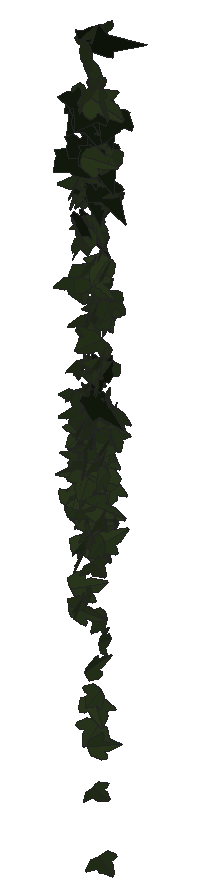
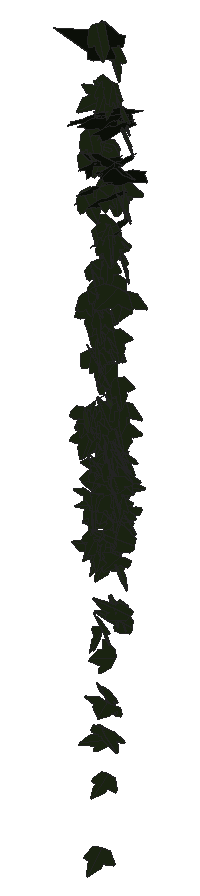
# SketchUp Ruby script. Lengths in inches.
U = 1.inch
M = Sketchup.active_model
def pt(a) = Geom::Point3d.new(a.map { |v| v * U })
def face(e, loops, mat)
  f = e.add_face(loops[0].map { |a| pt(a) })
  loops[1..].each { |l| e.add_face(l.map { |a| pt(a) }).erase! }
  f.material = f.back_material = mat if mat
  f
end
# faces: each face lists its corners as indices into pts; further lists are holes
def faces(e, pts, list, mat = nil) = list.each { |f| face(e, (f[0].is_a?(Array) ? f : [f]).map { |l| l.map { |i| pts[i] } }, mat) }
# xy, xz, yz: faces in a plane at the given z, y or x. An outline is a flat list of corners, or four numbers for a rectangle; further outlines are holes
def ring(l) = l.size == 4 ? [[l[0], l[1]], [l[2], l[1]], [l[2], l[3]], [l[0], l[3]]] : l.each_slice(2).to_a
def flat(e, list, mat, &to3) = list.each { |f| face(e, (f[0].is_a?(Array) ? f : [f]).map { |l| ring(l).map { |u, v| to3.(u, v) } }, mat) }
def xy(e, z, list, mat = nil) = flat(e, list, mat) { |x, y| [x, y, z] }
def xz(e, y, list, mat = nil) = flat(e, list, mat) { |x, z| [x, y, z] }
def yz(e, x, list, mat = nil) = flat(e, list, mat) { |y, z| [x, y, z] }
def lines(e, pts, list) = list.each { |a, b| e.add_line(pt(pts[a]), pt(pts[b])) }
# prism: a flat outline (further loops are holes) pulled along v
def prism(e, loops, v, mat = nil)
  f = face(e, loops, mat); d = Geom::Vector3d.new(v.map { |x| x * U })
  f.pushpull(f.normal.samedirection?(d) ? d.length : -d.length)
end
def box(e, o, s, mat = nil) = prism(e, [[o, [o[0] + s[0], o[1], o[2]], [o[0] + s[0], o[1] + s[1], o[2]], [o[0], o[1] + s[1], o[2]]]], [0, 0, s[2]], mat)
def at(x, y, z, deg = 0) = Geom::Transformation.translation(pt([x, y, z])) * Geom::Transformation.rotation(ORIGIN, Z_AXIS, deg.degrees)
def axes(o, x, y, z) = Geom::Transformation.new([*x, 0, *y, 0, *z, 0, *pt(o).to_a, 1])
def part(name) = M.definitions.add(name)
# library, detail: a bought-in or finely detailed component or shape, given as its bounding box
def library(name, o, s) = part(name).tap { |d| box(d.entities, o, s) }
def detail(e, o, s) = box(e.add_group.entities, o, s)
def put(e, d, t, mat = nil) = e.add_instance(d, t).tap { |i| i.material = mat if mat }
def group(e, t, mat = nil) = e.add_group.tap { |g| g.transformation = t; g.material = mat if mat }.entities
root = M.entities
M.materials.add("1026 AP 7946 SUNNY SIDE UP").color = [254, 231, 186]
M.materials.add("efeu1").color = [18, 25, 13]
M.materials.add("efeu2").color = [43, 57, 29]
c1 = part("ivyleaf_10")
p = [[0,0.5,-0.03],[-0.0625,2.02,-0.43],[-0.19,2.01,-0.46],[-0.54,1.05,-0.29],[-0.52,0.625,-0.18],[-0.83,0.76,-0.28],
  [-1.16,0.64,-0.33],[-1.15,0.33,-0.24],[-0.77,-0.39,0.02],[-0.3,-0.51,0.16],[0.04,-0.48,0.23],[-0.02,2.01,-0.4375],
  [-0.06,2.01,-0.43],[0.04,-0.49,0.23],[0.67,-0.49,0.14],[1.38,0.36,-0.2],[1.375,0.51,-0.24],[0.81,0.65,-0.19],
  [0.62,0.59,-0.15],[0.6,1.09,-0.28],[0.5,1.23,-0.31]]
faces(c1.entities,p,[[0,1,2,3,4,5,6,7,8,9,10],[11,12,0,13,14,15,16,17,18,19,20]],"efeu2")
c2 = part("ivyleaf_9")
p = [[1.54,2.16,1.25],[1.36,2.04,1.19],[-0.21,0.99,0.68],[-0.71,1.11,0.82],[-0.85,0.86,0.67],[-0.8,0.17,0.21],
  [-0.9,-0.01,0.1],[-0.67,-0.16,-0.02],[-0.08,-0.08,-0.05],[-0.03,-0.6,-0.4],[0.65,-0.88,-0.66],[0.83,-0.6,-0.49],
  [1.29,-0.42,-0.43],[1.8125,-0.07,-0.26],[1.21,0.44,0.15]]
faces(c2.entities,p,[[0,1,2,3,4,5,6,7,8,9,10,11,12,13,14]],"efeu1")
put(root,c1,axes([103.23,212.84,260.54],[-0.04694,-0.21641,-0.02736],[0.01178,0.02453,-0.22487],[0.3424,-0.03051,0.00399]),"1026 AP 7946 SUNNY SIDE UP")
put(root,c1,axes([103.25,212.84,259.06],[0.29938,-0.04666,-0.06917],[-0.11097,-0.00919,-0.20044],[0.06425,0.20159,-0.0239]),"1026 AP 7946 SUNNY SIDE UP")
put(root,c1,axes([103.31,212.77,258.55],[-0.28898,-0.07122,0.07311],[-0.08414,-0.05686,-0.20074],[0.13437,-0.18877,0.03152]),"1026 AP 7946 SUNNY SIDE UP")
put(root,c1,axes([103.3,212.68,263.19],[0.10199,-0.17927,-0.14312],[-0.09887,0.12352,-0.19515],[0.34162,0.08927,-0.01375]),"1026 AP 7946 SUNNY SIDE UP")
put(root,c1,axes([103.36,212.76,258.35],[0.02537,0.05885,-0.20622],[-0.24822,-0.12834,-0.05264],[-0.2153,0.1549,0.03639]),"1026 AP 7946 SUNNY SIDE UP")
put(root,c1,axes([103.25,212.75,259.54],[-0.16245,-0.19473,-0.00339],[0.01423,-0.00233,-0.22692],[0.30588,-0.10331,0.00875]),"1026 AP 7946 SUNNY SIDE UP")
put(root,c1,axes([103.28,212.8,258.09],[-0.26935,0.10482,0.02808],[-0.06448,-0.01673,-0.20375],[-0.15737,-0.17255,0.03542]),"1026 AP 7946 SUNNY SIDE UP")
put(root,c1,axes([103.26,212.6875,265.87],[0.2084,-0.21154,0.00222],[-0.01069,-0.00822,-0.257],[0.3325,0.13233,-0.00966]),"1026 AP 7946 SUNNY SIDE UP")
put(root,c1,axes([103.28,212.79,259.97],[-0.0656,-0.21468,-0.0423],[0.01333,0.03894,-0.22507],[0.34307,-0.04256,0.00066]),"1026 AP 7946 SUNNY SIDE UP")
put(root,c1,axes([103.24,212.68,262.31],[-0.2747,-0.15795,-0.04725],[0.07993,0.01042,-0.2411],[0.24556,-0.1801,0.02562]),"1026 AP 7946 SUNNY SIDE UP")
put(root,c1,axes([103.09,212.68,257.49],[0.16738,-0.12715,-0.14429],[0.16606,-0.0924,0.16944],[-0.24577,-0.14903,0.01622]),"1026 AP 7946 SUNNY SIDE UP")
put(root,c1,axes([103.3,212.59,264.51],[0.08272,-0.20959,-0.12985],[-0.0151,0.12585,-0.22107],[0.38331,0.05019,0.01931]),"1026 AP 7946 SUNNY SIDE UP")
put(root,c1,axes([103.26,212.86,259.22],[0.24489,-0.14597,0.00716],[-0.00431,-0.01428,-0.21961],[0.2298,0.15528,-0.01175]),"1026 AP 7946 SUNNY SIDE UP")
put(root,c1,axes([103.28,212.92,258.3],[0.1378,-0.1884,-0.00771],[0.00619,0.0089,-0.21388],[0.29635,0.08742,0.00805]),"1026 AP 7946 SUNNY SIDE UP")
put(root,c1,axes([103.4375,212.64,257.45],[0.25046,0.01853,0.16684],[-0.2547,0.04211,0.15951],[-0.02727,-0.22314,0.0426]),"1026 AP 7946 SUNNY SIDE UP")
put(root,c1,axes([103.27,212.9375,258.55],[0.27222,0.10499,-0.03679],[-0.04015,-0.02782,-0.20848],[-0.17,0.17469,-0.00967]),"1026 AP 7946 SUNNY SIDE UP")
put(root,c1,axes([103.3,212.72,257.41],[0.02496,-0.13732,-0.15549],[0.03087,0.15094,-0.13918],[0.31845,-0.00387,0.02568]),"1026 AP 7946 SUNNY SIDE UP")
put(root,c1,axes([103.05,212.86,257.27],[-0.03544,-0.04086,0.21982],[0.30269,0.0962,0.04044],[-0.15915,0.19206,0.02796]),"1026 AP 7946 SUNNY SIDE UP")
put(root,c1,axes([103.34,212.84,261.51],[-0.08217,-0.2236,0.00077],[0.00929,-0.00345,-0.23648],[0.35147,-0.05218,0.00643]),"1026 AP 7946 SUNNY SIDE UP")
put(root,c1,axes([103.3,212.68,257.78],[-0.10332,-0.18021,-0.08267],[0.06733,0.06844,-0.19656],[0.30212,-0.07688,0.01553]),"1026 AP 7946 SUNNY SIDE UP")
put(root,c1,axes([103.35,212.91,258.07],[-0.19602,-0.1599,0.04195],[0.01694,-0.05991,-0.20415],[0.25925,-0.11698,0.04506]),"1026 AP 7946 SUNNY SIDE UP")
put(root,c1,axes([103.35,212.67,266.32],[0.23053,-0.21398,-0.0296],[-0.02705,0.02157,-0.26709],[0.33816,0.1476,-0.00118]),"1026 AP 7946 SUNNY SIDE UP")
put(root,c1,axes([103.34,212.7,256.55],[0.11049,-0.19207,0.01732],[-0.00044,-0.01916,-0.21069],[0.30332,0.06994,-0.00661]),"1026 AP 7946 SUNNY SIDE UP")
put(root,c1,axes([103.34,212.67,264.38],[0.1732,-0.21768,0.02966],[0.00142,-0.03314,-0.2511],[0.34551,0.10926,-0.01384]),"1026 AP 7946 SUNNY SIDE UP")
put(root,c1,axes([103.36,212.63,259.94],[-0.34273,-0.04165,-0.0023],[0.00945,-0.02088,-0.22764],[0.06488,-0.21697,0.02102]),"1026 AP 7946 SUNNY SIDE UP")
put(root,c1,axes([103.27,212.5625,257.7],[0.24662,0.11259,-0.06619],[0.06847,0.0503,0.19862],[0.19253,-0.16212,0.01415]),"1026 AP 7946 SUNNY SIDE UP")
put(root,c1,axes([103.38,212.9,258.76],[-0.07272,-0.1991,0.054],[0.0002,-0.0549,-0.21052],[0.32419,-0.04463,0.01224]),"1026 AP 7946 SUNNY SIDE UP")
put(root,c1,axes([103.45,212.91,258.89],[-0.20192,0.13647,0.10363],[-0.14927,0.04553,-0.18967],[-0.22,-0.15614,0.03358]),"1026 AP 7946 SUNNY SIDE UP")
put(root,c1,axes([103.41,212.88,258.36],[-0.28504,-0.08988,0.02909],[-0.02468,-0.03266,-0.20739],[0.14631,-0.18061,0.02168]),"1026 AP 7946 SUNNY SIDE UP")
put(root,c1,axes([103.39,212.68,259.41],[0.11607,-0.21887,-0.03473],[-0.01485,0.03108,-0.23778],[0.34761,0.07441,0.00144]),"1026 AP 7946 SUNNY SIDE UP")
put(root,c1,axes([103.43,212.81,258.64],[-0.31976,-0.02335,0.02933],[-0.03642,-0.044,-0.20693],[0.04522,-0.20059,0.04073]),"1026 AP 7946 SUNNY SIDE UP")
put(root,c1,axes([103.39,212.92,263.53],[-0.15634,-0.21163,-0.00075],[0.03755,-0.01174,-0.23938],[0.33064,-0.09873,0.02683]),"1026 AP 7946 SUNNY SIDE UP")
put(root,c1,axes([103.41,212.59,255.64],[0.07677,-0.19731,-0.0096],[-0.00755,0.00726,-0.20933],[0.31043,0.04897,-0.00272]),"1026 AP 7946 SUNNY SIDE UP")
put(root,c2,axes([103.26,212.93,266.03],[-0.02722,-0.23947,-0.06366],[0.02114,0.05958,-0.24683],[0.38778,-0.02006,0.00899]),"1026 AP 7946 SUNNY SIDE UP")
put(root,c1,axes([103.15,212.84,255.74],[0.16252,-0.01027,-0.19384],[0.28883,0.05307,0.10131],[0.06568,-0.20796,0.03413]),"1026 AP 7946 SUNNY SIDE UP")
put(root,c2,axes([103.25,212.81,265.22],[0.07665,-0.22889,-0.08431],[-0.01243,0.08061,-0.24046],[0.38134,0.04863,0.00911]),"1026 AP 7946 SUNNY SIDE UP")
put(root,c2,axes([103.25,212.7,264.96],[-0.09652,-0.20028,-0.14831],[0.1107,0.12675,-0.21353],[0.37063,-0.09002,0.02515]),"1026 AP 7946 SUNNY SIDE UP")
put(root,c1,axes([103.3,212.92,262.5],[-0.29212,-0.08922,-0.10883],[0.17626,0.00501,-0.20841],[0.12626,-0.21341,0.03914]),"1026 AP 7946 SUNNY SIDE UP")
put(root,c1,axes([103.42,212.78,259.11],[-0.00647,-0.20589,-0.0613],[0.01607,0.05809,-0.21162],[0.3361,-0.00674,0.00894]),"1026 AP 7946 SUNNY SIDE UP")
put(root,c1,axes([103.4,212.92,266.8125],[-0.29063,0.15902,-0.0649],[-0.00392,-0.09647,-0.24045],[-0.26945,-0.17012,0.0735]),"1026 AP 7946 SUNNY SIDE UP")
put(root,c1,axes([103.63,212.54,263.31],[0.16098,-0.01365,0.23884],[-0.33599,0.09395,0.10342],[-0.14339,-0.23546,0.02581]),"1026 AP 7946 SUNNY SIDE UP")
put(root,c1,axes([103.45,212.93,259.1],[0.1097,-0.19976,-0.01619],[0.00222,0.01593,-0.21778],[0.31493,0.06947,0.00718]),"1026 AP 7946 SUNNY SIDE UP")
put(root,c1,axes([103.47,212.92,258.07],[-0.12624,-0.18476,0.04498],[0.00901,-0.05086,-0.20624],[0.29877,-0.07654,0.02523]),"1026 AP 7946 SUNNY SIDE UP")
put(root,c1,axes([103.53,212.6,264.53],[-0.32548,-0.17235,0.02063],[-0.00494,-0.02896,-0.27688],[0.27296,-0.20603,0.01959]),"1026 AP 7946 SUNNY SIDE UP")
put(root,c1,axes([103.32,212.78,256.8],[0.22563,0.11628,0.09147],[0.1297,0.0373,-0.18885],[-0.18923,0.16421,-0.02038]),"1026 AP 7946 SUNNY SIDE UP")
put(root,c1,axes([103.52,212.68,255.76],[0.11498,-0.17844,-0.07276],[-0.04144,0.06443,-0.19829],[0.29831,0.07773,0.0005]),"1026 AP 7946 SUNNY SIDE UP")
put(root,c1,axes([103.51,212.74,259.58],[-0.17421,-0.1843,-0.02236],[0.02661,0.01392,-0.22132],[0.2904,-0.11184,0.00687]),"1026 AP 7946 SUNNY SIDE UP")
put(root,c1,axes([103.55,212.59,267.38],[0.24893,-0.14422,-0.14549],[-0.07814,0.1451,-0.21041],[0.3067,0.15402,0.06448]),"1026 AP 7946 SUNNY SIDE UP")
put(root,c1,axes([103.52,212.56,256.95],[-0.00694,-0.19181,-0.08831],[0.00071,0.08465,-0.19716],[0.32966,-0.00422,-0.00143]),"1026 AP 7946 SUNNY SIDE UP")
put(root,c2,axes([103.67,213.01,265.28],[-0.37418,-0.02024,0.03644],[-0.05143,-0.03135,-0.24451],[0.0385,-0.23855,0.02761]),"1026 AP 7946 SUNNY SIDE UP")
put(root,c2,axes([103.54,212.73,266.16],[-0.26699,-0.17926,0.04318],[-0.02521,-0.04379,-0.25393],[0.28874,-0.16958,0.01776]),"1026 AP 7946 SUNNY SIDE UP")
put(root,c1,axes([103.56,212.7,263.55],[0.15078,-0.17246,-0.15179],[-0.04973,0.14719,-0.19915],[0.35218,0.09462,0.03686]),"1026 AP 7946 SUNNY SIDE UP")
put(root,c1,axes([103.24,212.65,255.39],[-0.02937,0.0052,0.22393],[0.33482,0.04441,0.01801],[-0.0689,0.21357,-0.0079]),"1026 AP 7946 SUNNY SIDE UP")
put(root,c1,axes([103.57,212.86,258.82],[-0.19139,-0.16572,0.02811],[-0.01067,-0.02997,-0.21163],[0.26411,-0.1213,0.01182]),"1026 AP 7946 SUNNY SIDE UP")
put(root,c1,axes([103.51,212.89,261.47],[0.26393,-0.15016,0.0086],[0.00225,-0.01219,-0.23193],[0.23654,0.16766,-0.00739]),"1026 AP 7946 SUNNY SIDE UP")
put(root,c1,axes([103.43,212.73,258.68],[0.1174,-0.13042,0.16058],[0.14206,-0.12833,-0.15522],[0.28727,0.11677,0.01113]),"1026 AP 7946 SUNNY SIDE UP")
put(root,c1,axes([103.57,212.78,263.65],[-0.13427,0.20039,0.09507],[-0.09339,0.07317,-0.22262],[-0.33332,-0.10122,0.02407]),"1026 AP 7946 SUNNY SIDE UP")
put(root,c1,axes([103.37,212.93,259.72],[-0.21302,0.05691,0.17785],[0.25355,-0.06088,0.15097],[0.13088,0.21057,-0.003]),"1026 AP 7946 SUNNY SIDE UP")
put(root,c1,axes([103.59,212.62,257.33],[-0.01236,0.0317,0.2202],[-0.11253,0.20125,-0.03231],[-0.3203,-0.07193,0.00285]),"1026 AP 7946 SUNNY SIDE UP")
put(root,c1,axes([103.76,212.74,259.53],[-0.22366,-0.00389,-0.16765],[-0.25389,0.03064,0.14483],[0.03229,0.21394,-0.02251]),"1026 AP 7946 SUNNY SIDE UP")
put(root,c2,axes([103.375,212.67,263.7],[0.21619,-0.1938,-0.06667],[-0.03483,0.06207,-0.24378],[0.31883,0.13819,0.01857]),"1026 AP 7946 SUNNY SIDE UP")
put(root,c1,axes([103.53,212.63,258.27],[0.35817,-0.01649,-0.01179],[-0.01974,-0.01666,-0.23468],[0.02453,0.22746,-0.0167]),"1026 AP 7946 SUNNY SIDE UP")
put(root,c1,axes([103.62,212.76,264.42],[-0.0404,-0.177,0.17265],[-0.02988,-0.16757,-0.18519],[0.3832,-0.03172,0.00376]),"1026 AP 7946 SUNNY SIDE UP")
put(root,c1,axes([103.53,212.72,260.07],[0.11903,-0.16028,0.13026],[0.06876,-0.11999,-0.18305],[0.31447,0.0869,-0.00928]),"1026 AP 7946 SUNNY SIDE UP")
put(root,c1,axes([103.6,212.89,258.625],[-0.1662,-0.18022,0.03375],[0.01314,-0.04369,-0.21341],[0.28801,-0.102,0.02922]),"1026 AP 7946 SUNNY SIDE UP")
put(root,c2,axes([103.44,212.69,265.95],[0.09263,-0.22441,-0.1139],[-0.05462,0.10382,-0.23832],[0.38867,0.06807,-0.00635]),"1026 AP 7946 SUNNY SIDE UP")
put(root,c1,axes([103.56,212.73,257.14],[-0.07492,-0.17846,-0.09029],[0.07353,0.07648,-0.18835],[0.30313,-0.06266,0.02337]),"1026 AP 7946 SUNNY SIDE UP")
put(root,c1,axes([103.8125,212.61,261.27],[-0.26726,-0.00474,0.17287],[-0.25522,-0.05643,-0.17132],[0.06751,-0.2321,0.03669]),"1026 AP 7946 SUNNY SIDE UP")
put(root,c1,axes([103.54,212.76,258.51],[0.03762,0.13375,0.16646],[0.00742,0.16148,-0.13814],[-0.32882,0.01895,0.01593]),"1026 AP 7946 SUNNY SIDE UP")
put(root,c1,axes([103.62,212.67,259.15],[0.02902,-0.19319,-0.10022],[0.0176,0.09727,-0.19848],[0.33889,0.01149,0.01889]),"1026 AP 7946 SUNNY SIDE UP")
put(root,c1,axes([103.61,212.8125,257.86],[-0.28311,0.09291,-0.00889],[0.00024,-0.0196,-0.20808],[-0.1468,-0.17922,0.0168]),"1026 AP 7946 SUNNY SIDE UP")
put(root,c1,axes([103.75,212.64,260.42],[-0.28214,0.08066,-0.10383],[-0.13214,0.05904,0.20223],[0.15482,0.19738,-0.01661]),"1026 AP 7946 SUNNY SIDE UP")
put(root,c1,axes([103.62,212.68,262.84],[-0.01732,-0.2207,-0.07356],[0.03598,0.06885,-0.22645],[0.36236,-0.01739,0.01897]),"1026 AP 7946 SUNNY SIDE UP")
put(root,c2,axes([103.5,212.83,264.39],[-0.02521,-0.24324,-0.02462],[0.01226,0.02205,-0.25092],[0.38391,-0.01668,0.0064]),"1026 AP 7946 SUNNY SIDE UP")
put(root,c1,axes([103.6,212.73,259.34],[-0.10218,-0.17317,-0.13413],[0.08172,0.11844,-0.18976],[0.32976,-0.08301,0.00546]),"1026 AP 7946 SUNNY SIDE UP")
put(root,c1,axes([103.88,212.72,259.09],[0.04926,0.00153,-0.23101],[-0.35107,0.02138,-0.03186],[0.03297,0.22541,0.00592]),"1026 AP 7946 SUNNY SIDE UP")
put(root,c1,axes([103.64,212.73,252.99],[0.3234,-0.0266,-0.03922],[-0.06285,-0.01477,-0.21279],[0.03679,0.20862,-0.01882]),"1026 AP 7946 SUNNY SIDE UP")
put(root,c1,axes([103.64,212.9375,259.28],[0.04506,0.16373,-0.13376],[-0.0622,-0.12539,-0.17139],[-0.32356,0.04691,0.01432]),"1026 AP 7946 SUNNY SIDE UP")
put(root,c1,axes([103.63,212.82,256.96],[-0.13553,-0.19424,-0.06788],[0.06726,0.05167,-0.21788],[0.31486,-0.09465,0.01732]),"1026 AP 7946 SUNNY SIDE UP")
put(root,c1,axes([103.68,212.81,261.79],[-0.05427,-0.21898,-0.07347],[0.01415,0.06952,-0.22796],[0.36125,-0.03562,-0.00211]),"1026 AP 7946 SUNNY SIDE UP")
put(root,c1,axes([103.6,212.84,258.83],[-0.10804,-0.16732,-0.10592],[0.12402,0.07519,-0.18159],[0.28196,-0.09719,0.03929]),"1026 AP 7946 SUNNY SIDE UP")
put(root,c1,axes([103.68,212.73,259.63],[-0.0611,-0.19059,-0.11073],[0.0465,0.10248,-0.19964],[0.34006,-0.04825,0.0074]),"1026 AP 7946 SUNNY SIDE UP")
put(root,c1,axes([103.66,212.65,266.56],[-0.06558,-0.23079,-0.15061],[0.09862,0.13451,-0.23854],[0.41698,-0.06811,0.03273]),"1026 AP 7946 SUNNY SIDE UP")
put(root,c1,axes([103.7,212.76,258.61],[-0.03221,-0.19677,-0.07565],[0.03693,0.07005,-0.2028],[0.32756,-0.02725,0.01542]),"1026 AP 7946 SUNNY SIDE UP")
put(root,c1,axes([103.75,212.8,267.81],[-0.08409,-0.25559,-0.01006],[-0.00015,0.00851,-0.26895],[0.4021,-0.05345,-0.0022]),"1026 AP 7946 SUNNY SIDE UP")
put(root,c1,axes([103.57,212.66,263.6875],[-0.27058,0.07127,-0.15087],[0.18309,-0.09596,-0.18909],[-0.17988,-0.20486,0.03448]),"1026 AP 7946 SUNNY SIDE UP")
put(root,c1,axes([103.75,212.63,253.79],[0.24642,-0.11789,-0.0533],[-0.08061,0.01647,-0.20116],[0.18523,0.164,-0.01665]),"1026 AP 7946 SUNNY SIDE UP")
put(root,c1,axes([103.52,212.56,257.41],[0.0218,-0.01516,0.23745],[0.18809,0.19811,0.00717],[-0.31087,0.1188,0.02099]),"1026 AP 7946 SUNNY SIDE UP")
put(root,c2,axes([103.59,212.9,266.05],[-0.04475,-0.23099,-0.08903],[0.0353,0.08288,-0.239],[0.38547,-0.03441,0.01155]),"1026 AP 7946 SUNNY SIDE UP")
put(root,c1,axes([103.68,212.91,258.6875],[0.3313,-0.00538,-0.00251],[-0.00455,-0.01959,-0.2163],[0.00808,0.2098,-0.01902]),"1026 AP 7946 SUNNY SIDE UP")
put(root,c1,axes([103.75,212.78,255.33],[0.21205,-0.15068,-0.04254],[-0.0545,0.02318,-0.20792],[0.23918,0.13887,-0.00967]),"1026 AP 7946 SUNNY SIDE UP")
put(root,c1,axes([103.57,212.77,266.49],[-0.21511,0.13896,-0.19272],[0.18263,-0.14846,-0.20113],[-0.31882,-0.1788,0.01482]),"1026 AP 7946 SUNNY SIDE UP")
put(root,c1,axes([103.76,212.71,258.05],[0.1358,-0.18241,-0.05248],[-0.02334,0.04816,-0.20751],[0.29644,0.08735,0.0077]),"1026 AP 7946 SUNNY SIDE UP")
put(root,c1,axes([103.78,212.82,262.38],[-0.06222,-0.22665,0.031],[-0.00243,-0.03158,-0.23717],[0.35977,-0.03941,0.00376]),"1026 AP 7946 SUNNY SIDE UP")
put(root,c1,axes([103.71,212.9,257.19],[-0.14754,-0.1634,-0.09792],[0.10114,0.0711,-0.19279],[0.27874,-0.11229,0.01812]),"1026 AP 7946 SUNNY SIDE UP")
put(root,c1,axes([103.82,212.9,259.87],[-0.13633,0.14005,0.13634],[-0.13,0.10308,-0.1686],[-0.27273,-0.11915,0.01221]),"1026 AP 7946 SUNNY SIDE UP")
put(root,c1,axes([103.7,212.84,261.9],[-0.337,0.03694,-0.07565],[0.09609,-0.06636,-0.21791],[-0.08688,-0.21669,0.05241]),"1026 AP 7946 SUNNY SIDE UP")
put(root,c1,axes([103.74,212.65,265.25],[-0.11321,-0.21649,-0.11993],[0.08583,0.10289,-0.23376],[0.37592,-0.08869,0.01725]),"1026 AP 7946 SUNNY SIDE UP")
put(root,c1,axes([103.82,212.95,259.52],[0.30911,0.00814,-0.08252],[-0.12566,0.04648,-0.19679],[0.01604,0.20715,0.04867]),"1026 AP 7946 SUNNY SIDE UP")
put(root,c1,axes([103.7,212.78,262.07],[0.02978,-0.10087,0.21686],[0.12323,-0.19679,-0.10528],[0.34659,0.07863,0.0188]),"1026 AP 7946 SUNNY SIDE UP")
put(root,c2,axes([103.63,212.83,265.11],[-0.01374,-0.23414,-0.0813],[0.03145,0.0767,-0.24035],[0.38657,-0.01456,0.01666]),"1026 AP 7946 SUNNY SIDE UP")
put(root,c1,axes([103.74,212.58,256.54],[-0.12641,-0.15871,-0.11217],[0.08774,0.09269,-0.1826],[0.2888,-0.09763,0.00638]),"1026 AP 7946 SUNNY SIDE UP")
put(root,c1,axes([103.79,212.82,262.84],[-0.15538,-0.1452,0.15402],[0.03683,-0.17293,-0.15722],[0.32657,-0.04958,0.09101]),"1026 AP 7946 SUNNY SIDE UP")
put(root,c1,axes([103.64,212.56,262.53],[-0.2105,-0.12947,-0.15642],[0.23341,0.0563,-0.18485],[0.20836,-0.19386,0.04905]),"1026 AP 7946 SUNNY SIDE UP")
put(root,c1,axes([103.8,212.83,261.89],[-0.3011,-0.12272,-0.01967],[0.03435,-0.00004,-0.234],[0.19208,-0.19237,0.01101]),"1026 AP 7946 SUNNY SIDE UP")
put(root,c1,axes([103.8,212.88,262.75],[0.10926,-0.22072,-0.02639],[0.01113,0.02772,-0.23772],[0.34899,0.06822,0.01584]),"1026 AP 7946 SUNNY SIDE UP")
put(root,c1,axes([103.83,212.94,265.63],[-0.08899,-0.23682,0.00602],[0.00754,-0.00854,-0.2508],[0.37247,-0.05641,0.00652]),"1026 AP 7946 SUNNY SIDE UP")
put(root,c1,axes([103.77,212.81,256.77],[0.00561,-0.18095,-0.1073],[0.06469,0.10172,-0.18181],[0.32103,-0.01734,0.03851]),"1026 AP 7946 SUNNY SIDE UP")
put(root,c1,axes([103.66,212.67,253.54],[0.29718,0.05485,0.07826],[0.12075,0.00609,-0.20215],[-0.08373,0.20348,-0.01376]),"1026 AP 7946 SUNNY SIDE UP")
put(root,c1,axes([103.85,212.6,257.01],[0.21159,-0.14812,-0.05761],[-0.06906,0.03444,-0.20575],[0.2387,0.14126,-0.00846]),"1026 AP 7946 SUNNY SIDE UP")
put(root,c1,axes([103.83,212.7,260.78],[-0.05747,-0.22608,-0.04214],[0.01603,0.03848,-0.23567],[0.36055,-0.03775,0.00376]),"1026 AP 7946 SUNNY SIDE UP")
put(root,c1,axes([103.74,212.97,258.77],[0.2543,-0.11292,0.06744],[0.0701,-0.05125,-0.20286],[0.19343,0.16703,-0.01514]),"1026 AP 7946 SUNNY SIDE UP")
put(root,c1,axes([103.8,212.43,254.38],[0.04432,-0.07994,0.22862],[-0.03858,0.22175,0.08662],[-0.36955,-0.03274,0.01838]),"1026 AP 7946 SUNNY SIDE UP")
put(root,c1,axes([103.93,212.8125,258.24],[0.05613,0.10492,0.17919],[-0.11622,-0.15714,0.11274],[0.29665,-0.08141,0.01027]),"1026 AP 7946 SUNNY SIDE UP")
put(root,c2,axes([104.01,212.51,260.57],[-0.04298,0.12481,0.22711],[-0.08491,0.21303,-0.13033],[-0.38819,-0.06041,0.00336]),"1026 AP 7946 SUNNY SIDE UP")
put(root,c1,axes([103.95,212.83,257.63],[-0.16545,0.11649,0.13258],[-0.16873,0.07367,-0.15947],[-0.21357,-0.14845,0.02328]),"1026 AP 7946 SUNNY SIDE UP")
put(root,c1,axes([103.89,212.64,254.9],[-0.00758,0.05166,0.20218],[-0.12672,0.17936,-0.04971],[-0.29237,-0.07908,0.0163]),"1026 AP 7946 SUNNY SIDE UP")
put(root,c1,axes([103.74,212.47,265.18],[0.04141,0.10665,0.24039],[0.06339,0.22932,-0.11161],[-0.39753,0.04768,0.00724]),"1026 AP 7946 SUNNY SIDE UP")
put(root,c1,axes([103.75,212.75,260.37],[-0.00932,-0.00034,0.23154],[0.17283,-0.19612,0.00154],[0.30826,0.10994,0.00614]),"1026 AP 7946 SUNNY SIDE UP")
put(root,c1,axes([103.87,212.95,259.71],[0.03972,-0.20622,0.03433],[0.00463,-0.03439,-0.21423],[0.32873,0.0254,-0.00113]),"1026 AP 7946 SUNNY SIDE UP")
put(root,c1,axes([103.88,212.72,263.36],[0.13424,-0.22557,-0.03318],[-0.01322,0.02989,-0.24827],[0.35776,0.08575,0.00327]),"1026 AP 7946 SUNNY SIDE UP")
put(root,c1,axes([103.77,212.96,258.06],[0.3147,0.01696,0.02967],[0.04797,-0.02278,-0.20544],[-0.02112,0.2009,-0.02461]),"1026 AP 7946 SUNNY SIDE UP")
put(root,c1,axes([103.9,212.87,262.16],[-0.15752,-0.19474,0.07333],[0.00837,-0.08264,-0.22222],[0.32652,-0.09183,0.04108]),"1026 AP 7946 SUNNY SIDE UP")
put(root,c1,axes([103.96,212.64,260.81],[-0.24166,-0.14623,0.07872],[-0.05579,-0.07383,-0.21716],[0.25398,-0.15535,0.02719]),"1026 AP 7946 SUNNY SIDE UP")
put(root,c1,axes([103.9,212.64,258.93],[0.0979,-0.18559,-0.09621],[-0.01788,0.0932,-0.20035],[0.32545,0.06095,0.01793]),"1026 AP 7946 SUNNY SIDE UP")
put(root,c1,axes([103.91,212.73,259.12],[0.06546,-0.21122,-0.04812],[-0.02452,0.04329,-0.22142],[0.33886,0.04394,-0.00672]),"1026 AP 7946 SUNNY SIDE UP")
put(root,c1,axes([103.83,212.49,251.83],[-0.11326,-0.13714,-0.13504],[0.10899,0.1106,-0.15874],[0.27677,-0.09968,0.00725]),"1026 AP 7946 SUNNY SIDE UP")
put(root,c1,axes([103.98,212.64,261.82],[0.15859,-0.16106,-0.1331],[-0.12573,0.101,-0.19481],[0.29836,0.12817,-0.01135]),"1026 AP 7946 SUNNY SIDE UP")
put(root,c2,axes([103.72,212.52,260.08],[0.20051,-0.15692,-0.1381],[-0.04993,0.13977,-0.20019],[0.31973,0.12023,0.05534]),"1026 AP 7946 SUNNY SIDE UP")
put(root,c1,axes([103.91,212.57,260.99],[0.02771,-0.20412,-0.09247],[0.00023,0.08889,-0.21042],[0.34989,0.01611,0.00746]),"1026 AP 7946 SUNNY SIDE UP")
put(root,c1,axes([103.89,212.61,257.54],[-0.00459,-0.18336,-0.09923],[0.04116,0.09419,-0.18701],[0.32229,-0.01464,0.02247]),"1026 AP 7946 SUNNY SIDE UP")
put(root,c1,axes([103.88,212.91,259.23],[-0.2627,-0.11788,-0.05074],[0.07063,0.02052,-0.21033],[0.18763,-0.17277,0.00814]),"1026 AP 7946 SUNNY SIDE UP")
put(root,c1,axes([103.95,212.76,262.02],[-0.21943,-0.18009,0.03075],[-0.01104,-0.03353,-0.23441],[0.28709,-0.13894,0.01449]),"1026 AP 7946 SUNNY SIDE UP")
put(root,c1,axes([103.65,212.61,257.74],[0.06671,0.05124,0.22653],[0.26684,0.13989,-0.06658],[-0.23348,0.17451,-0.01137]),"1026 AP 7946 SUNNY SIDE UP")
put(root,c1,axes([103.8,212.54,252.71],[-0.00591,-0.00038,0.22063],[0.07166,0.20929,0.00244],[-0.32904,0.04559,-0.00343]),"1026 AP 7946 SUNNY SIDE UP")
put(root,c1,axes([103.76,212.81,256.91],[0.10529,0.06159,-0.2206],[0.20069,0.17312,0.09327],[0.28783,-0.14324,0.01567]),"1026 AP 7946 SUNNY SIDE UP")
put(root,c1,axes([103.7,212.59,266.37],[0.17469,0.14069,0.21442],[0.18247,0.17213,-0.18337],[-0.34919,0.16033,0.01145]),"1026 AP 7946 SUNNY SIDE UP")
put(root,c1,axes([103.86,212.63,250.3],[-0.14247,-0.17433,-0.1083],[0.11093,0.07991,-0.20058],[0.29941,-0.11256,0.02278]),"1026 AP 7946 SUNNY SIDE UP")
put(root,c1,axes([103.94,212.84,265.18],[-0.14121,-0.20112,0.10904],[0.0132,-0.11784,-0.22165],[0.35796,-0.075,0.05119]),"1026 AP 7946 SUNNY SIDE UP")
put(root,c1,axes([103.97,212.88,264.26],[-0.07169,-0.23107,0.05835],[-0.02172,-0.05634,-0.24295],[0.37395,-0.04757,-0.00293]),"1026 AP 7946 SUNNY SIDE UP")
put(root,c2,axes([103.59,212.69,267.5],[0.13559,0.00832,0.25253],[0.38548,-0.00907,-0.0886],[0.00912,0.25965,-0.00967]),"1026 AP 7946 SUNNY SIDE UP")
put(root,c1,axes([103.94,212.6,258.5],[0.22439,-0.14655,-0.03358],[-0.04862,0.01415,-0.21028],[0.23073,0.14551,-0.01165]),"1026 AP 7946 SUNNY SIDE UP")
put(root,c2,axes([103.75,212.78,264.51],[0.06191,-0.2176,-0.11031],[0.0267,0.10946,-0.22467],[0.37954,0.0278,0.0338]),"1026 AP 7946 SUNNY SIDE UP")
put(root,c2,axes([103.89,213.02,266.02],[-0.16347,-0.21277,0.0652],[-0.00751,-0.06905,-0.24298],[0.34951,-0.101,0.02528]),"1026 AP 7946 SUNNY SIDE UP")
put(root,c1,axes([103.96,212.95,259.7],[-0.30426,0.0877,0.01867],[-0.03372,-0.00471,-0.21847],[-0.13656,-0.19425,0.01236]),"1026 AP 7946 SUNNY SIDE UP")
